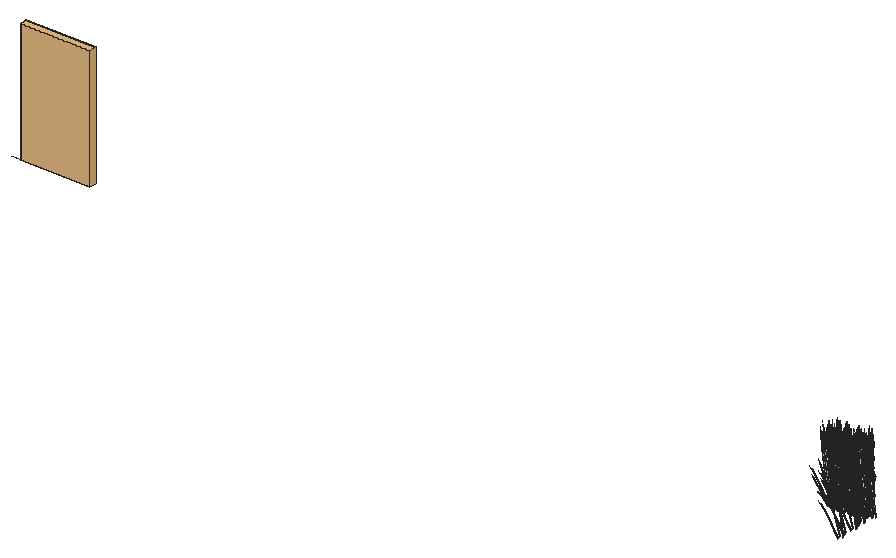
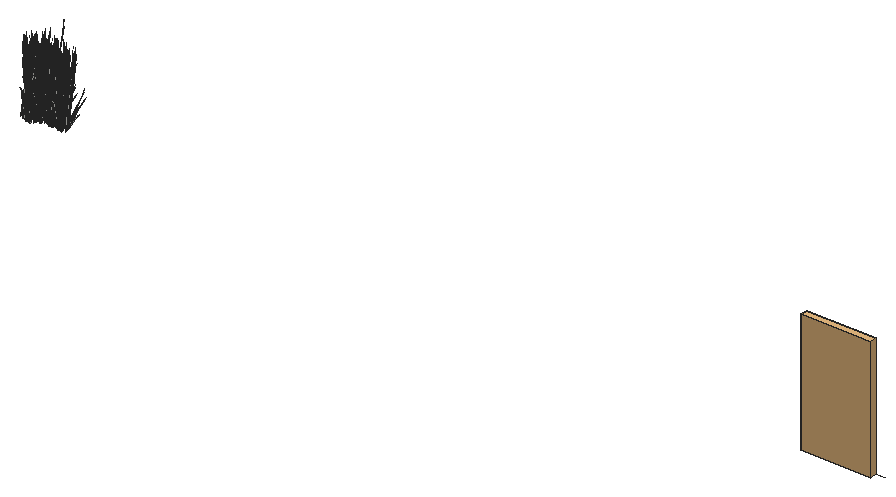
# SketchUp Ruby script. Lengths in inches.
U = 1.inch
M = Sketchup.active_model
def pt(a) = Geom::Point3d.new(a.map { |v| v * U })
def face(e, loops, mat)
  f = e.add_face(loops[0].map { |a| pt(a) })
  loops[1..].each { |l| e.add_face(l.map { |a| pt(a) }).erase! }
  f.material = f.back_material = mat if mat
  f
end
# faces: each face lists its corners as indices into pts; further lists are holes
def faces(e, pts, list, mat = nil) = list.each { |f| face(e, (f[0].is_a?(Array) ? f : [f]).map { |l| l.map { |i| pts[i] } }, mat) }
# xy, xz, yz: faces in a plane at the given z, y or x. An outline is a flat list of corners, or four numbers for a rectangle; further outlines are holes
def ring(l) = l.size == 4 ? [[l[0], l[1]], [l[2], l[1]], [l[2], l[3]], [l[0], l[3]]] : l.each_slice(2).to_a
def flat(e, list, mat, &to3) = list.each { |f| face(e, (f[0].is_a?(Array) ? f : [f]).map { |l| ring(l).map { |u, v| to3.(u, v) } }, mat) }
def xy(e, z, list, mat = nil) = flat(e, list, mat) { |x, y| [x, y, z] }
def xz(e, y, list, mat = nil) = flat(e, list, mat) { |x, z| [x, y, z] }
def yz(e, x, list, mat = nil) = flat(e, list, mat) { |y, z| [x, y, z] }
def lines(e, pts, list) = list.each { |a, b| e.add_line(pt(pts[a]), pt(pts[b])) }
# prism: a flat outline (further loops are holes) pulled along v
def prism(e, loops, v, mat = nil)
  f = face(e, loops, mat); d = Geom::Vector3d.new(v.map { |x| x * U })
  f.pushpull(f.normal.samedirection?(d) ? d.length : -d.length)
end
def box(e, o, s, mat = nil) = prism(e, [[o, [o[0] + s[0], o[1], o[2]], [o[0] + s[0], o[1] + s[1], o[2]], [o[0], o[1] + s[1], o[2]]]], [0, 0, s[2]], mat)
def at(x, y, z, deg = 0) = Geom::Transformation.translation(pt([x, y, z])) * Geom::Transformation.rotation(ORIGIN, Z_AXIS, deg.degrees)
def axes(o, x, y, z) = Geom::Transformation.new([*x, 0, *y, 0, *z, 0, *pt(o).to_a, 1])
def part(name) = M.definitions.add(name)
# library, detail: a bought-in or finely detailed component or shape, given as its bounding box
def library(name, o, s) = part(name).tap { |d| box(d.entities, o, s) }
def detail(e, o, s) = box(e.add_group.entities, o, s)
def put(e, d, t, mat = nil) = e.add_instance(d, t).tap { |i| i.material = mat if mat }
def group(e, t, mat = nil) = e.add_group.tap { |g| g.transformation = t; g.material = mat if mat }.entities
root = M.entities
M.materials.add("LightPink_Translucent").color = [144, 107, 117]
M.materials["LightPink_Translucent"].alpha = 0.75
c1 = library("porta+4",[0.2,-5.42,1.33],[46.55,4.72,83.21])
c2 = part("blade")
p = [[2.15,0.21,22],[0,0.17,0],[0.09,0.45,0],[2.18,0.31,22],[2.29,0.31,22],[0.38,0.45,0],
  [2.48,0.24,33],[2.49,0.24,33],[2.48,0.22,33]]
faces(c2.entities,p,[[0,1,2,3],[4,5,2,3],[6,3,4,7],[8,0,3,6]])
c3 = part("seeds")
p = [[0.3,-0.1,1.38],[-0.01,-0.03,1.59],[-0.01,-0.03,0.03],[0.14,-0.07,-0.07],[0.29,-0.03,3],[0.15,0.01,3.11]]
faces(c3.entities,p,[[0,1,2,3],[1,0,4,5]],"LightPink_Translucent")
c4 = part("blade with seeds")
put(c4.entities,c2,at(0,0,0))
put(c4.entities,c3,axes([2.4,0.25,30.99],[1.5799,-0.05474,1.17369],[-0.12525,1.92788,0.29478],[-0.07173,-0.02425,1.56792]))
p = [[75,360,266],[81,360,266]]
lines(root,p,[[0,1]])
put(root,c1,axes([129.21,359.3,264.66],[-1.03118,0,0],[0,-1,0],[0,0,1.00971]))
put(root,c4,axes([656.875,338.03,266.15],[0.2261,0.04687,1.18691],[0.14573,0.47875,-0.25526],[-0.30712,0.08962,0.50747]))
put(root,c4,axes([657.75,335.72,266.15],[0.12702,0.15896,1.18691],[-0.2927,0.4321,-0.25526],[-0.30054,-0.10328,0.50747]))
put(root,c4,axes([656.4,339.04,266.3],[0.27113,-0.25877,0.95334],[0.10699,0.40966,0.70045],[-0.19594,0.07335,0.20998]))
put(root,c4,axes([656.99,336.19,266.3],[0.41536,-0.04086,0.95334],[-0.26347,0.35999,0.70045],[-0.20525,-0.054,0.20998]))
put(root,c4,axes([658.95,339.04,265.97],[-0.40676,0.57214,0],[-0.68052,-0.31907,-0.42834],[-0.15499,-0.07267,1.3588]))
put(root,c4,axes([658.21,339.86,266.15],[0.2053,-0.09007,1.18691],[0.50689,0.27159,-0.25526],[-0.15087,0.235,0.50747]))
put(root,c4,axes([658.78,334.14,266.15],[-0.0394,0.18678,1.18691],[-0.57594,0.15636,-0.25526],[-0.13463,-0.24142,0.50747]))
put(root,c4,axes([657.61,336.86,265.97],[-0.81352,0,0],[0,-0.63814,-0.42834],[0,-0.14534,1.3588]))
put(root,c4,axes([658.24,336.6875,265.93],[-0.60515,0.48003,0.25528],[-0.60552,-0.47498,-0.30288],[-0.02113,-0.13632,1.36855]))
put(root,c4,axes([658.58,333.84,266.3],[0.33937,0.19872,0.95334],[-0.49424,0.11946,0.70045],[-0.10575,-0.15273,0.20998]))
put(root,c4,axes([658.7,340.17,266.3],[-0.01684,-0.3395,0.95334],[0.42072,0.24214,0.70045],[-0.08274,0.16182,0.20998]))
put(root,c4,axes([659.3,338.74,266.06],[0.60889,0.28548,0.4121],[-0.36394,0.51192,0],[-0.13868,-0.06502,1.30728]))
put(root,c4,axes([660.18,337.85,266.17],[-0.12551,0.50956,0.12018],[-0.6132,-0.08845,-0.34318],[-0.1116,-0.05232,1.05198]))
put(root,c4,axes([658.1,336.95,266.06],[0,0.57097,0.4121],[-0.72788,0,0],[0,-0.13004,1.30728]))
put(root,c4,axes([661.4375,339.11,265.82],[-0.40169,-0.57414,-0.04268],[0.68052,-0.31907,0.42834],[-0.16769,0.05466,1.35813]))
put(root,c4,axes([663.58,337.5,266.15],[0.2261,0.04687,1.18691],[0.14573,0.47875,-0.25526],[-0.30712,0.08962,0.50747]))
put(root,c4,axes([658.35,339.43,266.34],[0.59102,-0.10111,0.05401],[0.13587,0.40735,-0.71633],[-0.03747,0.2062,0.64209]))
put(root,c4,axes([659.97,337.36,265.96],[0.82229,0.1203,0.37976],[-0.16734,0.67942,0.14902],[-0.12017,-0.06561,1.31851]))
put(root,c4,axes([664.45,335.18,266.15],[0.12702,0.15896,1.18691],[-0.2927,0.4321,-0.25526],[-0.30054,-0.10328,0.50747]))
put(root,c4,axes([659.76,337.24,266.26],[-0.31565,0.51449,0.37133],[-0.65588,-0.24761,-0.17871],[0,-0.1186,1.19224]))
put(root,c4,axes([659.53,338.45,266.05],[0.6991,-0.15154,0.14643],[0.17263,0.56398,0.29122],[-0.06235,-0.08217,1.33138]))
put(root,c4,axes([660.43,338.54,265.82],[-0.65588,-0.25634,0],[0.31565,-0.53263,0],[0,0,1.35047]))
put(root,c4,axes([661.95,339.18,265.97],[0.40676,0.57214,0],[-0.68052,0.31907,-0.42834],[-0.15499,0.07267,1.3588]))
put(root,c4,axes([661.61,338.48,266.05],[0.18794,-0.56744,0.14643],[0.68774,0.16058,0.29122],[-0.1188,0.00276,1.33138]))
put(root,c4,axes([661.29,337.73,266.17],[0.48065,0.34305,0.12018],[-0.40092,0.38703,-0.34318],[-0.1116,0.05232,1.05198]))
put(root,c4,axes([663.11,338.5,266.3],[0.27113,-0.25877,0.95334],[0.10699,0.40966,0.70045],[-0.19594,0.07335,0.20998]))
put(root,c4,axes([661.125,337.3,265.91],[-0.60515,-0.49144,-0.05089],[0.60552,-0.49174,0],[-0.02113,-0.01716,1.45724]))
put(root,c4,axes([661.28,337.47,266.26],[0.70648,-0.03525,0.37133],[0.06389,0.58508,-0.17871],[-0.12647,0.0593,1.19224]))
put(root,c4,axes([661.45,338.82,265.93],[0.81449,0.18558,0.25528],[-0.20377,0.66335,-0.30288],[-0.13481,0.08302,1.36855]))
put(root,c4,axes([661.81,338.78,266.06],[0.60889,-0.28548,0.4121],[0.36394,0.51192,0],[-0.13868,0.06502,1.30728]))
put(root,c4,axes([659.9,336.74,265.96],[0.28286,0.63846,0.37976],[-0.80821,0.22202,0.14902],[0.00988,-0.11732,1.31851]))
put(root,c4,axes([660.58,338.32,265.83],[-0.21227,-0.49226,0],[0.60616,-0.17239,0],[0,0,1.28128]))
put(root,c4,axes([663.7,335.66,266.3],[0.41536,-0.04086,0.95334],[-0.26347,0.35999,0.70045],[-0.20525,-0.054,0.20998]))
put(root,c4,axes([662.6875,337.03,266.05],[-0.51116,-0.4159,0.14643],[0.51512,-0.4034,0.29122],[-0.05645,0.08494,1.33138]))
put(root,c4,axes([660.92,336.79,265.83],[0,-0.66065,0],[0.81352,0,0],[0,0,1.48949]))
put(root,c4,axes([660.16,336.91,266.02],[0.73304,0.27674,0.19974],[-0.35279,0.57501,0.41502],[0,-0.13255,1.3325]))
put(root,c4,axes([661.33,337.06,265.9],[0,0.66033,-0.04679],[-0.81352,0,0],[0,0.02075,1.48875]))
put(root,c4,axes([659.93,336.53,266.26],[-0.70648,0.03525,0.37133],[-0.06389,-0.58508,-0.17871],[0.12647,-0.0593,1.19224]))
put(root,c4,axes([659.6,335.52,266.05],[-0.18794,0.56744,0.14643],[-0.68774,-0.16058,0.29122],[0.1188,-0.00276,1.33138]))
put(root,c4,axes([660.94,338.33,265.9],[0.28286,0.65594,-0.0499],[-0.80821,0.22985,0],[0.00988,0.02291,1.42904]))
put(root,c4,axes([659.26,334.82,265.97],[-0.40676,-0.57214,0],[0.68052,-0.31907,-0.42834],[0.15499,-0.07267,1.3588]))
put(root,c4,axes([663.28,337.47,265.83],[-0.81312,-0.00457,-0.0413],[0,-0.63814,0.41452],[-0.02555,0.14527,1.31432]))
put(root,c4,axes([661.68,335.55,266.05],[-0.6991,0.15154,0.14643],[-0.17263,-0.56398,0.29122],[0.06235,0.08217,1.33138]))
put(root,c4,axes([660.96,333.4375,266.3],[0.08346,0.33295,0.95334],[-0.46298,-0.1844,0.70045],[0.04982,-0.17048,0.20998]))
put(root,c4,axes([660.53,336.375,265.96],[-0.53943,0.51816,0.37976],[-0.64086,-0.4574,0.14902],[0.13005,-0.05171,1.31851]))
put(root,c4,axes([661.46,337.19,265.84],[0.45414,0.3688,0],[-0.45414,0.3688,0],[0,0,1.40491]))
put(root,c4,axes([661.45,336.76,266.26],[0.31565,-0.51449,0.37133],[0.65588,0.24761,-0.17871],[0,0.1186,1.19224]))
put(root,c4,axes([661.18,338.55,265.83],[0.65588,0.25634,0],[-0.31565,0.53263,0],[0,0,1.45212]))
put(root,c4,axes([665.66,338.5,265.97],[-0.40676,0.57214,0],[-0.68052,-0.31907,-0.42834],[-0.15499,-0.07267,1.3588]))
put(root,c4,axes([661.24,336.64,265.98],[-0.82229,-0.1203,0.40835],[0.16734,-0.67942,0.16024],[0.12017,0.06561,1.41775]))
put(root,c4,axes([661.47,336.9375,265.83],[0.72788,0,0],[0,0.59111,0],[0,0,1.48078]))
put(root,c4,axes([664.92,339.33,266.15],[0.2053,-0.09007,1.18691],[0.50689,0.27159,-0.25526],[-0.15087,0.235,0.50747]))
put(root,c4,axes([660.77,336.29,266.26],[-0.39083,-0.47924,0.37133],[0.59199,-0.33747,-0.17871],[0.12647,0.0593,1.19224]))
put(root,c4,axes([661.72,336.88,266.17],[0.60616,-0.16651,0.12018],[0.21227,0.47548,-0.34318],[0,0.10465,1.05198]))
put(root,c4,axes([665.49,333.61,266.15],[-0.0394,0.18678,1.18691],[-0.57594,0.15636,-0.25526],[-0.13463,-0.24142,0.50747]))
put(root,c4,axes([661.65,334.36,266.15],[-0.18493,0.11557,1.18691],[-0.55384,-0.20228,-0.25526],[0.10266,-0.25157,0.50747]))
put(root,c4,axes([664.3125,336.32,265.97],[-0.81352,0,0],[0,-0.63814,-0.42834],[0,-0.14534,1.3588]))
put(root,c4,axes([663.11,337.05,266.06],[0,-0.57097,0.4121],[0.72788,0,0],[0,0.13004,1.30728]))
put(root,c4,axes([661.03,336.15,266.17],[0.12551,-0.50956,0.12018],[0.6132,0.08845,-0.34318],[0.1116,0.05232,1.05198]))
put(root,c4,axes([664.94,336.15,265.93],[-0.60515,0.48003,0.25528],[-0.60552,-0.47498,-0.30288],[-0.02113,-0.13632,1.36855]))
put(root,c4,axes([661.91,335.26,266.06],[-0.60889,-0.28548,0.4121],[0.36394,-0.51192,0],[0.13868,0.06502,1.30728]))
put(root,c4,axes([665.29,333.3,266.3],[0.33937,0.19872,0.95334],[-0.49424,0.11946,0.70045],[-0.10575,-0.15273,0.20998]))
put(root,c4,axes([665.41,339.63,266.3],[-0.01684,-0.3395,0.95334],[0.42072,0.24214,0.70045],[-0.08274,0.16182,0.20998]))
put(root,c4,axes([666.01,338.2,266.06],[0.60889,0.28548,0.4121],[-0.36394,0.51192,0],[-0.13868,-0.06502,1.30728]))
put(root,c4,axes([662.49,338.76,266.3],[-0.36631,-0.16417,0.95334],[0.47299,-0.16681,0.70045],[0.12758,0.1413,0.20998]))
put(root,c4,axes([661.19,338.59,266.15],[0.01148,-0.18927,1.18691],[0.54864,-0.21141,-0.25526],[0.16937,0.22654,0.50747]))
put(root,c4,axes([666.88,337.3125,266.17],[-0.12551,0.50956,0.12018],[-0.6132,-0.08845,-0.34318],[-0.1116,-0.05232,1.05198]))
put(root,c4,axes([664.81,336.42,266.06],[0,0.57097,0.4121],[-0.72788,0,0],[0,-0.13004,1.30728]))
put(root,c4,axes([668.14,338.58,265.82],[-0.40169,-0.57414,-0.04268],[0.68052,-0.31907,0.42834],[-0.16769,0.05466,1.35813]))
put(root,c4,axes([663.6,337.14,265.97],[0.81352,0,0],[0,0.63814,-0.42834],[0,0.14534,1.3588]))
put(root,c4,axes([662.55,339.51,266.21],[-0.4172,-0.01791,0.872],[0.27552,-0.38032,0.48145],[0.16481,0.13512,0.68401]))
put(root,c4,axes([665.06,338.9,266.34],[0.59102,-0.10111,0.05401],[0.13587,0.40735,-0.71633],[-0.03747,0.2062,0.64209]))
put(root,c4,axes([666.68,336.83,265.96],[0.82229,0.1203,0.37976],[-0.16734,0.67942,0.14902],[-0.12017,-0.06561,1.31851]))
put(root,c4,axes([662.26,334.97,265.97],[0.40676,-0.57214,0],[0.68052,0.31907,-0.42834],[0.15499,0.07267,1.3588]))
put(root,c4,axes([666.46,336.71,266.26],[-0.31565,0.51449,0.37133],[-0.65588,-0.24761,-0.17871],[0,-0.1186,1.19224]))
put(root,c4,axes([666.24,337.91,266.05],[0.6991,-0.15154,0.14643],[0.17263,0.56398,0.29122],[-0.06235,-0.08217,1.33138]))
put(root,c4,axes([667.14,338,265.82],[-0.65588,-0.25634,0],[0.31565,-0.53263,0],[0,0,1.35047]))
put(root,c4,axes([671.48,338.09,266.15],[0.2261,0.04687,1.18691],[0.14573,0.47875,-0.25526],[-0.30712,0.08962,0.50747]))
put(root,c4,axes([668.65,338.64,265.97],[0.40676,0.57214,0],[-0.68052,0.31907,-0.42834],[-0.15499,0.07267,1.3588]))
put(root,c4,axes([668.32,337.94,266.05],[0.18794,-0.56744,0.14643],[0.68774,0.16058,0.29122],[-0.1188,0.00276,1.33138]))
put(root,c4,axes([663.69,334.89,266.3],[-0.2167,0.29065,0.95334],[-0.18626,-0.3905,0.70045],[0.17898,-0.09785,0.20998]))
put(root,c4,axes([668,337.19,266.17],[0.48065,0.34305,0.12018],[-0.40092,0.38703,-0.34318],[-0.1116,0.05232,1.05198]))
put(root,c4,axes([667.83,336.77,265.91],[-0.60515,-0.49144,-0.05089],[0.60552,-0.49174,0],[-0.02113,-0.01716,1.45724]))
put(root,c4,axes([667.99,336.94,266.26],[0.70648,-0.03525,0.37133],[0.06389,0.58508,-0.17871],[-0.12647,0.0593,1.19224]))
put(root,c4,axes([668.16,338.29,265.93],[0.81449,0.18558,0.25528],[-0.20377,0.66335,-0.30288],[-0.13481,0.08302,1.36855]))
put(root,c4,axes([668.51,338.25,266.06],[0.60889,-0.28548,0.4121],[0.36394,0.51192,0],[-0.13868,0.06502,1.30728]))
put(root,c4,axes([666.61,336.2,265.96],[0.28286,0.63846,0.37976],[-0.80821,0.22202,0.14902],[0.00988,-0.11732,1.31851]))
put(root,c4,axes([672.35,335.78,266.15],[0.12702,0.15896,1.18691],[-0.2927,0.4321,-0.25526],[-0.30054,-0.10328,0.50747]))
put(root,c4,axes([667.29,337.78,265.83],[-0.21227,-0.49226,0],[0.60616,-0.17239,0],[0,0,1.28128]))
put(root,c4,axes([669.39,336.5,266.05],[-0.51116,-0.4159,0.14643],[0.51512,-0.4034,0.29122],[-0.05645,0.08494,1.33138]))
put(root,c4,axes([667.625,336.26,265.83],[0,-0.66065,0],[0.81352,0,0],[0,0,1.48949]))
put(root,c4,axes([666.87,336.375,266.02],[0.73304,0.27674,0.19974],[-0.35279,0.57501,0.41502],[0,-0.13255,1.3325]))
put(root,c4,axes([668.03,336.52,265.9],[0,0.66033,-0.04679],[-0.81352,0,0],[0,0.02075,1.48875]))
put(root,c4,axes([671.01,339.1,266.3],[0.27113,-0.25877,0.95334],[0.10699,0.40966,0.70045],[-0.19594,0.07335,0.20998]))
put(root,c4,axes([666.63,335.99,266.26],[-0.70648,0.03525,0.37133],[-0.06389,-0.58508,-0.17871],[0.12647,-0.0593,1.19224]))
put(root,c4,axes([666.3,334.99,266.05],[-0.18794,0.56744,0.14643],[-0.68774,-0.16058,0.29122],[0.1188,-0.00276,1.33138]))
put(root,c4,axes([664.73,337.41,266.3],[-0.40197,0.09426,0.95334],[0.18921,-0.38956,0.70045],[0.21325,0.02666,0.20998]))
put(root,c4,axes([667.64,337.8,265.9],[0.28286,0.65594,-0.0499],[-0.80821,0.22985,0],[0.00988,0.02291,1.42904]))
put(root,c4,axes([663.43,335.72,266.15],[-0.23242,-0.01691,1.18691],[-0.23811,-0.45367,-0.25526],[0.28553,-0.12834,0.50747]))
put(root,c4,axes([665.97,334.29,265.97],[-0.40676,-0.57214,0],[0.68052,-0.31907,-0.42834],[0.15499,-0.07267,1.3588]))
put(root,c4,axes([669.98,336.9375,265.83],[-0.81312,-0.00457,-0.0413],[0,-0.63814,0.41452],[-0.02555,0.14527,1.31432]))
put(root,c4,axes([671.6,336.25,266.3],[0.41536,-0.04086,0.95334],[-0.26347,0.35999,0.70045],[-0.20525,-0.054,0.20998]))
put(root,c4,axes([668.38,335.02,266.05],[-0.6991,0.15154,0.14643],[-0.17263,-0.56398,0.29122],[0.06235,0.08217,1.33138]))
put(root,c4,axes([667.67,332.9,266.3],[0.08346,0.33295,0.95334],[-0.46298,-0.1844,0.70045],[0.04982,-0.17048,0.20998]))
put(root,c4,axes([667.24,335.84,265.96],[-0.53943,0.51816,0.37976],[-0.64086,-0.4574,0.14902],[0.13005,-0.05171,1.31851]))
put(root,c4,axes([668.16,336.66,265.84],[0.45414,0.3688,0],[-0.45414,0.3688,0],[0,0,1.40491]))
put(root,c4,axes([668.15,336.23,266.26],[0.31565,-0.51449,0.37133],[0.65588,0.24761,-0.17871],[0,0.1186,1.19224]))
put(root,c4,axes([667.88,338.01,265.83],[0.65588,0.25634,0],[-0.31565,0.53263,0],[0,0,1.45212]))
put(root,c4,axes([667.94,336.1,265.98],[-0.82229,-0.1203,0.40835],[0.16734,-0.67942,0.16024],[0.12017,0.06561,1.41775]))
put(root,c4,axes([668.18,336.4,265.83],[0.72788,0,0],[0,0.59111,0],[0,0,1.48078]))
put(root,c4,axes([667.48,335.75,266.26],[-0.39083,-0.47924,0.37133],[0.59199,-0.33747,-0.17871],[0.12647,0.0593,1.19224]))
put(root,c4,axes([668.43,336.34,266.17],[0.60616,-0.16651,0.12018],[0.21227,0.47548,-0.34318],[0,0.10465,1.05198]))
put(root,c4,axes([663.98,338.04,266.15],[-0.15668,-0.14043,1.18691],[0.20386,-0.46454,-0.25526],[0.31701,0.06293,0.50747]))
put(root,c4,axes([668.35,333.82,266.15],[-0.18493,0.11557,1.18691],[-0.55384,-0.20228,-0.25526],[0.10266,-0.25157,0.50747]))
put(root,c4,axes([669.8125,336.51,266.06],[0,-0.57097,0.4121],[0.72788,0,0],[0,0.13004,1.30728]))
put(root,c4,axes([673.56,339.09,265.97],[-0.40676,0.57214,0],[-0.68052,-0.31907,-0.42834],[-0.15499,-0.07267,1.3588]))
put(root,c4,axes([667.74,335.62,266.17],[0.12551,-0.50956,0.12018],[0.6132,0.08845,-0.34318],[0.1116,0.05232,1.05198]))
put(root,c4,axes([668.61,334.73,266.06],[-0.60889,-0.28548,0.4121],[0.36394,-0.51192,0],[0.13868,0.06502,1.30728]))
put(root,c4,axes([672.82,339.92,266.15],[0.2053,-0.09007,1.18691],[0.50689,0.27159,-0.25526],[-0.15087,0.235,0.50747]))
put(root,c4,axes([673.39,334.2,266.15],[-0.0394,0.18678,1.18691],[-0.57594,0.15636,-0.25526],[-0.13463,-0.24142,0.50747]))
put(root,c4,axes([672.21,336.92,265.97],[-0.81352,0,0],[0,-0.63814,-0.42834],[0,-0.14534,1.3588]))
put(root,c4,axes([676.28,341.16,266.15],[0.2261,0.04687,1.18691],[0.14573,0.47875,-0.25526],[-0.30712,0.08962,0.50747]))
put(root,c4,axes([669.2,338.23,266.3],[-0.36631,-0.16417,0.95334],[0.47299,-0.16681,0.70045],[0.12758,0.1413,0.20998]))
put(root,c4,axes([667.89,338.05,266.15],[0.01148,-0.18927,1.18691],[0.54864,-0.21141,-0.25526],[0.16937,0.22654,0.50747]))
put(root,c4,axes([672.84,336.75,265.93],[-0.60515,0.48003,0.25528],[-0.60552,-0.47498,-0.30288],[-0.02113,-0.13632,1.36855]))
put(root,c4,axes([670.31,336.61,265.97],[0.81352,0,0],[0,0.63814,-0.42834],[0,0.14534,1.3588]))
put(root,c4,axes([673.1875,333.9,266.3],[0.33937,0.19872,0.95334],[-0.49424,0.11946,0.70045],[-0.10575,-0.15273,0.20998]))
put(root,c4,axes([669.26,338.97,266.21],[-0.4172,-0.01791,0.872],[0.27552,-0.38032,0.48145],[0.16481,0.13512,0.68401]))
put(root,c4,axes([677.15,338.85,266.15],[0.12702,0.15896,1.18691],[-0.2927,0.4321,-0.25526],[-0.30054,-0.10328,0.50747]))
put(root,c4,axes([673.31,340.22,266.3],[-0.01684,-0.3395,0.95334],[0.42072,0.24214,0.70045],[-0.08274,0.16182,0.20998]))
put(root,c4,axes([673.91,338.8,266.06],[0.60889,0.28548,0.4121],[-0.36394,0.51192,0],[-0.13868,-0.06502,1.30728]))
put(root,c4,axes([674.78,337.91,266.17],[-0.12551,0.50956,0.12018],[-0.6132,-0.08845,-0.34318],[-0.1116,-0.05232,1.05198]))
put(root,c4,axes([668.96,334.43,265.97],[0.40676,-0.57214,0],[0.68052,0.31907,-0.42834],[0.15499,0.07267,1.3588]))
put(root,c4,axes([672.71,337.01,266.06],[0,0.57097,0.4121],[-0.72788,0,0],[0,-0.13004,1.30728]))
put(root,c4,axes([676.04,339.17,265.82],[-0.40169,-0.57414,-0.04268],[0.68052,-0.31907,0.42834],[-0.16769,0.05466,1.35813]))
put(root,c4,axes([675.81,342.17,266.3],[0.27113,-0.25877,0.95334],[0.10699,0.40966,0.70045],[-0.19594,0.07335,0.20998]))
put(root,c4,axes([672.96,339.49,266.34],[0.59102,-0.10111,0.05401],[0.13587,0.40735,-0.71633],[-0.03747,0.2062,0.64209]))
put(root,c4,axes([676.4,339.32,266.3],[0.41536,-0.04086,0.95334],[-0.26347,0.35999,0.70045],[-0.20525,-0.054,0.20998]))
put(root,c4,axes([670.4,334.35,266.3],[-0.2167,0.29065,0.95334],[-0.18626,-0.3905,0.70045],[0.17898,-0.09785,0.20998]))
put(root,c4,axes([674.58,337.42,265.96],[0.82229,0.1203,0.37976],[-0.16734,0.67942,0.14902],[-0.12017,-0.06561,1.31851]))
put(root,c4,axes([674.37,337.3,266.26],[-0.31565,0.51449,0.37133],[-0.65588,-0.24761,-0.17871],[0,-0.1186,1.19224]))
put(root,c4,axes([674.14,338.51,266.05],[0.6991,-0.15154,0.14643],[0.17263,0.56398,0.29122],[-0.06235,-0.08217,1.33138]))
put(root,c4,axes([675.04,338.6,265.82],[-0.65588,-0.25634,0],[0.31565,-0.53263,0],[0,0,1.35047]))
put(root,c4,axes([676.55,339.24,265.97],[0.40676,0.57214,0],[-0.68052,0.31907,-0.42834],[-0.15499,0.07267,1.3588]))
put(root,c4,axes([676.22,338.54,266.05],[0.18794,-0.56744,0.14643],[0.68774,0.16058,0.29122],[-0.1188,0.00276,1.33138]))
put(root,c4,axes([675.9,337.79,266.17],[0.48065,0.34305,0.12018],[-0.40092,0.38703,-0.34318],[-0.1116,0.05232,1.05198]))
put(root,c4,axes([675.73,337.36,265.91],[-0.60515,-0.49144,-0.05089],[0.60552,-0.49174,0],[-0.02113,-0.01716,1.45724]))
put(root,c4,axes([675.89,337.53,266.26],[0.70648,-0.03525,0.37133],[0.06389,0.58508,-0.17871],[-0.12647,0.0593,1.19224]))
put(root,c4,axes([676.06,338.88,265.93],[0.81449,0.18558,0.25528],[-0.20377,0.66335,-0.30288],[-0.13481,0.08302,1.36855]))
put(root,c4,axes([671.43,336.875,266.3],[-0.40197,0.09426,0.95334],[0.18921,-0.38956,0.70045],[0.21325,0.02666,0.20998]))
put(root,c4,axes([678.36,342.17,265.97],[-0.40676,0.57214,0],[-0.68052,-0.31907,-0.42834],[-0.15499,-0.07267,1.3588]))
put(root,c4,axes([676.41,338.84,266.06],[0.60889,-0.28548,0.4121],[0.36394,0.51192,0],[-0.13868,0.06502,1.30728]))
put(root,c4,axes([670.13,335.18,266.15],[-0.23242,-0.01691,1.18691],[-0.23811,-0.45367,-0.25526],[0.28553,-0.12834,0.50747]))
put(root,c4,axes([674.51,336.8,265.96],[0.28286,0.63846,0.37976],[-0.80821,0.22202,0.14902],[0.00988,-0.11732,1.31851]))
put(root,c4,axes([675.1875,338.375,265.83],[-0.21227,-0.49226,0],[0.60616,-0.17239,0],[0,0,1.28128]))
put(root,c4,axes([677.62,342.99,266.15],[0.2053,-0.09007,1.18691],[0.50689,0.27159,-0.25526],[-0.15087,0.235,0.50747]))
put(root,c4,axes([678.1875,337.27,266.15],[-0.0394,0.18678,1.18691],[-0.57594,0.15636,-0.25526],[-0.13463,-0.24142,0.50747]))
put(root,c4,axes([677.29,337.09,266.05],[-0.51116,-0.4159,0.14643],[0.51512,-0.4034,0.29122],[-0.05645,0.08494,1.33138]))
put(root,c4,axes([675.52,336.85,265.83],[0,-0.66065,0],[0.81352,0,0],[0,0,1.48949]))
put(root,c4,axes([674.77,336.97,266.02],[0.73304,0.27674,0.19974],[-0.35279,0.57501,0.41502],[0,-0.13255,1.3325]))
put(root,c4,axes([675.93,337.11,265.9],[0,0.66033,-0.04679],[-0.81352,0,0],[0,0.02075,1.48875]))
put(root,c4,axes([674.53,336.59,266.26],[-0.70648,0.03525,0.37133],[-0.06389,-0.58508,-0.17871],[0.12647,-0.0593,1.19224]))
put(root,c4,axes([677.02,339.99,265.97],[-0.81352,0,0],[0,-0.63814,-0.42834],[0,-0.14534,1.3588]))
put(root,c4,axes([674.2,335.58,266.05],[-0.18794,0.56744,0.14643],[-0.68774,-0.16058,0.29122],[0.1188,-0.00276,1.33138]))
put(root,c4,axes([675.54,338.39,265.9],[0.28286,0.65594,-0.0499],[-0.80821,0.22985,0],[0.00988,0.02291,1.42904]))
put(root,c4,axes([673.87,334.88,265.97],[-0.40676,-0.57214,0],[0.68052,-0.31907,-0.42834],[0.15499,-0.07267,1.3588]))
put(root,c4,axes([670.68,337.5,266.15],[-0.15668,-0.14043,1.18691],[0.20386,-0.46454,-0.25526],[0.31701,0.06293,0.50747]))
put(root,c4,axes([677.88,337.53,265.83],[-0.81312,-0.00457,-0.0413],[0,-0.63814,0.41452],[-0.02555,0.14527,1.31432]))
put(root,c4,axes([677.65,339.82,265.93],[-0.60515,0.48003,0.25528],[-0.60552,-0.47498,-0.30288],[-0.02113,-0.13632,1.36855]))
put(root,c4,axes([676.28,335.61,266.05],[-0.6991,0.15154,0.14643],[-0.17263,-0.56398,0.29122],[0.06235,0.08217,1.33138]))
put(root,c4,axes([677.99,336.97,266.3],[0.33937,0.19872,0.95334],[-0.49424,0.11946,0.70045],[-0.10575,-0.15273,0.20998]))
put(root,c4,axes([675.57,333.5,266.3],[0.08346,0.33295,0.95334],[-0.46298,-0.1844,0.70045],[0.04982,-0.17048,0.20998]))
put(root,c4,axes([681.71,339.62,266.15],[0.2261,0.04687,1.18691],[0.14573,0.47875,-0.25526],[-0.30712,0.08962,0.50747]))
put(root,c4,axes([675.14,336.43,265.96],[-0.53943,0.51816,0.37976],[-0.64086,-0.4574,0.14902],[0.13005,-0.05171,1.31851]))
put(root,c4,axes([676.0625,337.25,265.84],[0.45414,0.3688,0],[-0.45414,0.3688,0],[0,0,1.40491]))
put(root,c4,axes([676.05,336.82,266.26],[0.31565,-0.51449,0.37133],[0.65588,0.24761,-0.17871],[0,0.1186,1.19224]))
put(root,c4,axes([675.78,338.61,265.83],[0.65588,0.25634,0],[-0.31565,0.53263,0],[0,0,1.45212]))
put(root,c4,axes([678.11,343.3,266.3],[-0.01684,-0.3395,0.95334],[0.42072,0.24214,0.70045],[-0.08274,0.16182,0.20998]))
put(root,c4,axes([675.84,336.7,265.98],[-0.82229,-0.1203,0.40835],[0.16734,-0.67942,0.16024],[0.12017,0.06561,1.41775]))
put(root,c4,axes([678.71,341.87,266.06],[0.60889,0.28548,0.4121],[-0.36394,0.51192,0],[-0.13868,-0.06502,1.30728]))
put(root,c4,axes([676.08,337,265.83],[0.72788,0,0],[0,0.59111,0],[0,0,1.48078]))
put(root,c4,axes([675.375,336.35,266.26],[-0.39083,-0.47924,0.37133],[0.59199,-0.33747,-0.17871],[0.12647,0.0593,1.19224]))
put(root,c4,axes([676.33,336.9375,266.17],[0.60616,-0.16651,0.12018],[0.21227,0.47548,-0.34318],[0,0.10465,1.05198]))
put(root,c4,axes([679.58,340.98,266.17],[-0.12551,0.50956,0.12018],[-0.6132,-0.08845,-0.34318],[-0.1116,-0.05232,1.05198]))
put(root,c4,axes([682.58,337.3,266.15],[0.12702,0.15896,1.18691],[-0.2927,0.4321,-0.25526],[-0.30054,-0.10328,0.50747]))
put(root,c4,axes([677.51,340.08,266.06],[0,0.57097,0.4121],[-0.72788,0,0],[0,-0.13004,1.30728]))
put(root,c4,axes([680.84,342.25,265.82],[-0.40169,-0.57414,-0.04268],[0.68052,-0.31907,0.42834],[-0.16769,0.05466,1.35813]))
put(root,c4,axes([676.25,334.42,266.15],[-0.18493,0.11557,1.18691],[-0.55384,-0.20228,-0.25526],[0.10266,-0.25157,0.50747]))
put(root,c4,axes([683.05,331.43,266.15],[0.2261,0.04687,1.18691],[0.14573,0.47875,-0.25526],[-0.30712,0.08962,0.50747]))
put(root,c4,axes([677.71,337.11,266.06],[0,-0.57097,0.4121],[0.72788,0,0],[0,0.13004,1.30728]))
put(root,c4,axes([677.76,342.5625,266.34],[0.59102,-0.10111,0.05401],[0.13587,0.40735,-0.71633],[-0.03747,0.2062,0.64209]))
put(root,c4,axes([675.64,336.21,266.17],[0.12551,-0.50956,0.12018],[0.6132,0.08845,-0.34318],[0.1116,0.05232,1.05198]))
put(root,c4,axes([681.23,340.625,266.3],[0.27113,-0.25877,0.95334],[0.10699,0.40966,0.70045],[-0.19594,0.07335,0.20998]))
put(root,c4,axes([676.51,335.32,266.06],[-0.60889,-0.28548,0.4121],[0.36394,-0.51192,0],[0.13868,0.06502,1.30728]))
put(root,c4,axes([679.38,340.49,265.96],[0.82229,0.1203,0.37976],[-0.16734,0.67942,0.14902],[-0.12017,-0.06561,1.31851]))
put(root,c4,axes([679.17,340.37,266.26],[-0.31565,0.51449,0.37133],[-0.65588,-0.24761,-0.17871],[0,-0.1186,1.19224]))
put(root,c4,axes([683.92,329.12,266.15],[0.12702,0.15896,1.18691],[-0.2927,0.4321,-0.25526],[-0.30054,-0.10328,0.50747]))
put(root,c4,axes([681.82,337.78,266.3],[0.41536,-0.04086,0.95334],[-0.26347,0.35999,0.70045],[-0.20525,-0.054,0.20998]))
put(root,c4,axes([678.9375,341.58,266.05],[0.6991,-0.15154,0.14643],[0.17263,0.56398,0.29122],[-0.06235,-0.08217,1.33138]))
put(root,c4,axes([684.1,323.23,266.15],[0.2261,0.04687,1.18691],[0.14573,0.47875,-0.25526],[-0.30712,0.08962,0.50747]))
put(root,c4,axes([684.13,311.75,266.15],[0.2261,0.04687,1.18691],[0.14573,0.47875,-0.25526],[-0.30712,0.08962,0.50747]))
put(root,c4,axes([679.84,341.67,265.82],[-0.65588,-0.25634,0],[0.31565,-0.53263,0],[0,0,1.35047]))
put(root,c4,axes([677.1,338.82,266.3],[-0.36631,-0.16417,0.95334],[0.47299,-0.16681,0.70045],[0.12758,0.1413,0.20998]))
put(root,c4,axes([675.8,338.65,266.15],[0.01148,-0.18927,1.18691],[0.54864,-0.21141,-0.25526],[0.16937,0.22654,0.50747]))
put(root,c4,axes([681.35,342.31,265.97],[0.40676,0.57214,0],[-0.68052,0.31907,-0.42834],[-0.15499,0.07267,1.3588]))
put(root,c4,axes([681.02,341.61,266.05],[0.18794,-0.56744,0.14643],[0.68774,0.16058,0.29122],[-0.1188,0.00276,1.33138]))
put(root,c4,axes([680.7,340.86,266.17],[0.48065,0.34305,0.12018],[-0.40092,0.38703,-0.34318],[-0.1116,0.05232,1.05198]))
put(root,c4,axes([684.56,316.69,266.15],[0.2261,0.04687,1.18691],[0.14573,0.47875,-0.25526],[-0.30712,0.08962,0.50747]))
put(root,c4,axes([678.21,337.2,265.97],[0.81352,0,0],[0,0.63814,-0.42834],[0,0.14534,1.3588]))
put(root,c4,axes([680.53,340.43,265.91],[-0.60515,-0.49144,-0.05089],[0.60552,-0.49174,0],[-0.02113,-0.01716,1.45724]))
put(root,c4,axes([680.6875,340.6,266.26],[0.70648,-0.03525,0.37133],[0.06389,0.58508,-0.17871],[-0.12647,0.0593,1.19224]))
put(root,c4,axes([682.57,332.4375,266.3],[0.27113,-0.25877,0.95334],[0.10699,0.40966,0.70045],[-0.19594,0.07335,0.20998]))
put(root,c4,axes([680.86,341.95,265.93],[0.81449,0.18558,0.25528],[-0.20377,0.66335,-0.30288],[-0.13481,0.08302,1.36855]))
put(root,c4,axes([677.16,339.57,266.21],[-0.4172,-0.01791,0.872],[0.27552,-0.38032,0.48145],[0.16481,0.13512,0.68401]))
put(root,c4,axes([681.21,341.91,266.06],[0.60889,-0.28548,0.4121],[0.36394,0.51192,0],[-0.13868,0.06502,1.30728]))
put(root,c4,axes([684.97,320.92,266.15],[0.12702,0.15896,1.18691],[-0.2927,0.4321,-0.25526],[-0.30054,-0.10328,0.50747]))
put(root,c4,axes([685.01,309.43,266.15],[0.12702,0.15896,1.18691],[-0.2927,0.4321,-0.25526],[-0.30054,-0.10328,0.50747]))
put(root,c4,axes([679.31,339.87,265.96],[0.28286,0.63846,0.37976],[-0.80821,0.22202,0.14902],[0.00988,-0.11732,1.31851]))
put(root,c4,axes([679.99,341.45,265.83],[-0.21227,-0.49226,0],[0.60616,-0.17239,0],[0,0,1.28128]))
put(root,c4,axes([683.16,329.59,266.3],[0.41536,-0.04086,0.95334],[-0.26347,0.35999,0.70045],[-0.20525,-0.054,0.20998]))
put(root,c4,axes([685.43,314.375,266.15],[0.12702,0.15896,1.18691],[-0.2927,0.4321,-0.25526],[-0.30054,-0.10328,0.50747]))
put(root,c4,axes([683.78,340.62,265.97],[-0.40676,0.57214,0],[-0.68052,-0.31907,-0.42834],[-0.15499,-0.07267,1.3588]))
put(root,c4,axes([676.86,335.03,265.97],[0.40676,-0.57214,0],[0.68052,0.31907,-0.42834],[0.15499,0.07267,1.3588]))
put(root,c4,axes([682.09,340.16,266.05],[-0.51116,-0.4159,0.14643],[0.51512,-0.4034,0.29122],[-0.05645,0.08494,1.33138]))
put(root,c4,axes([680.33,339.92,265.83],[0,-0.66065,0],[0.81352,0,0],[0,0,1.48949]))
put(root,c4,axes([679.57,340.04,266.02],[0.73304,0.27674,0.19974],[-0.35279,0.57501,0.41502],[0,-0.13255,1.3325]))
put(root,c4,axes([680.73,340.19,265.9],[0,0.66033,-0.04679],[-0.81352,0,0],[0,0.02075,1.48875]))
put(root,c4,axes([679.33,339.66,266.26],[-0.70648,0.03525,0.37133],[-0.06389,-0.58508,-0.17871],[0.12647,-0.0593,1.19224]))
put(root,c4,axes([683.04,341.45,266.15],[0.2053,-0.09007,1.18691],[0.50689,0.27159,-0.25526],[-0.15087,0.235,0.50747]))
put(root,c4,axes([679,338.65,266.05],[-0.18794,0.56744,0.14643],[-0.68774,-0.16058,0.29122],[0.1188,-0.00276,1.33138]))
put(root,c4,axes([680.35,341.46,265.9],[0.28286,0.65594,-0.0499],[-0.80821,0.22985,0],[0.00988,0.02291,1.42904]))
put(root,c4,axes([683.61,335.73,266.15],[-0.0394,0.18678,1.18691],[-0.57594,0.15636,-0.25526],[-0.13463,-0.24142,0.50747]))
put(root,c4,axes([678.67,337.95,265.97],[-0.40676,-0.57214,0],[0.68052,-0.31907,-0.42834],[0.15499,-0.07267,1.3588]))
put(root,c4,axes([682.68,340.6,265.83],[-0.81312,-0.00457,-0.0413],[0,-0.63814,0.41452],[-0.02555,0.14527,1.31432]))
put(root,c4,axes([681.08,338.68,266.05],[-0.6991,0.15154,0.14643],[-0.17263,-0.56398,0.29122],[0.06235,0.08217,1.33138]))
put(root,c4,axes([678.3,334.95,266.3],[-0.2167,0.29065,0.95334],[-0.18626,-0.3905,0.70045],[0.17898,-0.09785,0.20998]))
put(root,c4,axes([682.44,338.44,265.97],[-0.81352,0,0],[0,-0.63814,-0.42834],[0,-0.14534,1.3588]))
put(root,c4,axes([680.37,336.57,266.3],[0.08346,0.33295,0.95334],[-0.46298,-0.1844,0.70045],[0.04982,-0.17048,0.20998]))
put(root,c4,axes([679.94,339.51,265.96],[-0.53943,0.51816,0.37976],[-0.64086,-0.4574,0.14902],[0.13005,-0.05171,1.31851]))
put(root,c4,axes([680.86,340.32,265.84],[0.45414,0.3688,0],[-0.45414,0.3688,0],[0,0,1.40491]))
put(root,c4,axes([680.86,339.89,266.26],[0.31565,-0.51449,0.37133],[0.65588,0.24761,-0.17871],[0,0.1186,1.19224]))
put(root,c4,axes([680.58,341.68,265.83],[0.65588,0.25634,0],[-0.31565,0.53263,0],[0,0,1.45212]))
put(root,c4,axes([685.125,332.43,265.97],[-0.40676,0.57214,0],[-0.68052,-0.31907,-0.42834],[-0.15499,-0.07267,1.3588]))
put(root,c4,axes([680.64,339.77,265.98],[-0.82229,-0.1203,0.40835],[0.16734,-0.67942,0.16024],[0.12017,0.06561,1.41775]))
put(root,c4,axes([683.07,338.28,265.93],[-0.60515,0.48003,0.25528],[-0.60552,-0.47498,-0.30288],[-0.02113,-0.13632,1.36855]))
put(root,c4,axes([683.42,335.43,266.3],[0.33937,0.19872,0.95334],[-0.49424,0.11946,0.70045],[-0.10575,-0.15273,0.20998]))
put(root,c4,axes([680.88,340.07,265.83],[0.72788,0,0],[0,0.59111,0],[0,0,1.48078]))
put(root,c4,axes([680.18,339.42,266.26],[-0.39083,-0.47924,0.37133],[0.59199,-0.33747,-0.17871],[0.12647,0.0593,1.19224]))
put(root,c4,axes([681.13,340.01,266.17],[0.60616,-0.16651,0.12018],[0.21227,0.47548,-0.34318],[0,0.10465,1.05198]))
put(root,c4,axes([684.38,333.26,266.15],[0.2053,-0.09007,1.18691],[0.50689,0.27159,-0.25526],[-0.15087,0.235,0.50747]))
put(root,c4,axes([683.53,341.75,266.3],[-0.01684,-0.3395,0.95334],[0.42072,0.24214,0.70045],[-0.08274,0.16182,0.20998]))
put(root,c4,axes([684.95,327.54,266.15],[-0.0394,0.18678,1.18691],[-0.57594,0.15636,-0.25526],[-0.13463,-0.24142,0.50747]))
put(root,c4,axes([684.14,340.32,266.06],[0.60889,0.28548,0.4121],[-0.36394,0.51192,0],[-0.13868,-0.06502,1.30728]))
put(root,c4,axes([681.05,337.49,266.15],[-0.18493,0.11557,1.18691],[-0.55384,-0.20228,-0.25526],[0.10266,-0.25157,0.50747]))
put(root,c4,axes([683.78,330.26,265.97],[-0.81352,0,0],[0,-0.63814,-0.42834],[0,-0.14534,1.3588]))
put(root,c4,axes([686.18,324.23,265.97],[-0.40676,0.57214,0],[-0.68052,-0.31907,-0.42834],[-0.15499,-0.07267,1.3588]))
put(root,c4,axes([679.33,337.47,266.3],[-0.40197,0.09426,0.95334],[0.18921,-0.38956,0.70045],[0.21325,0.02666,0.20998]))
put(root,c4,axes([682.51,340.18,266.06],[0,-0.57097,0.4121],[0.72788,0,0],[0,0.13004,1.30728]))
put(root,c4,axes([685.01,339.4375,266.17],[-0.12551,0.50956,0.12018],[-0.6132,-0.08845,-0.34318],[-0.1116,-0.05232,1.05198]))
put(root,c4,axes([686.21,312.75,265.97],[-0.40676,0.57214,0],[-0.68052,-0.31907,-0.42834],[-0.15499,-0.07267,1.3588]))
put(root,c4,axes([680.44,339.28,266.17],[0.12551,-0.50956,0.12018],[0.6132,0.08845,-0.34318],[0.1116,0.05232,1.05198]))
put(root,c4,axes([682.93,338.54,266.06],[0,0.57097,0.4121],[-0.72788,0,0],[0,-0.13004,1.30728]))
put(root,c4,axes([686.27,340.7,265.82],[-0.40169,-0.57414,-0.04268],[0.68052,-0.31907,0.42834],[-0.16769,0.05466,1.35813]))
put(root,c4,axes([678.03,335.78,266.15],[-0.23242,-0.01691,1.18691],[-0.23811,-0.45367,-0.25526],[0.28553,-0.12834,0.50747]))
put(root,c4,axes([681.3125,338.39,266.06],[-0.60889,-0.28548,0.4121],[0.36394,-0.51192,0],[0.13868,0.06502,1.30728]))
